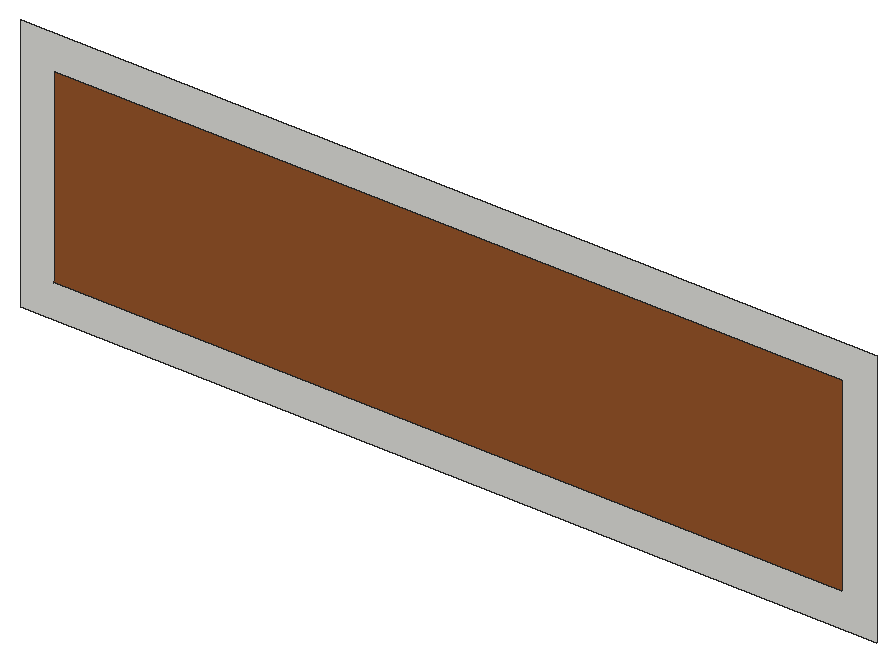
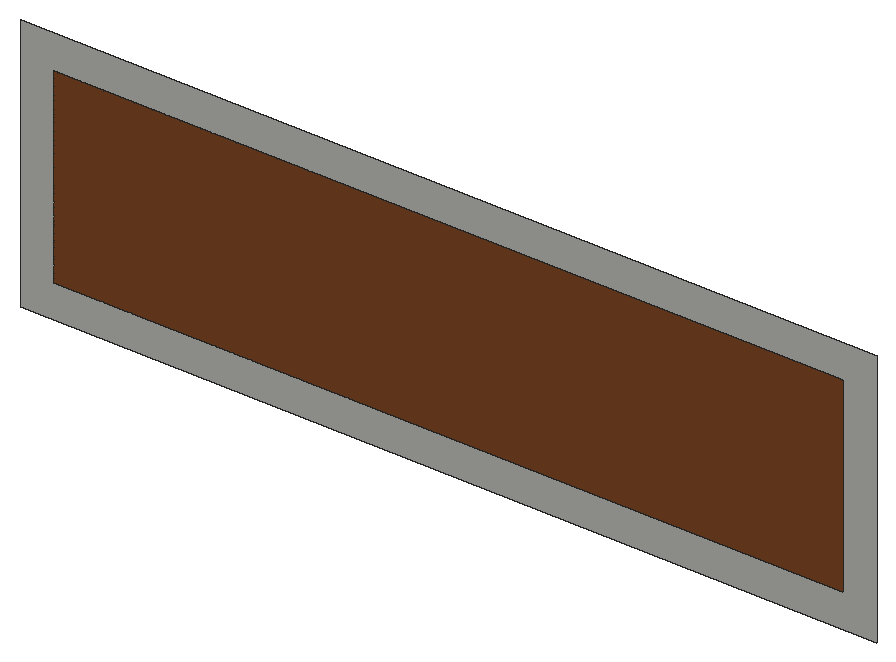
# SketchUp Ruby script. Lengths in inches.
U = 1.inch
M = Sketchup.active_model
def pt(a) = Geom::Point3d.new(a.map { |v| v * U })
def face(e, loops, mat)
  f = e.add_face(loops[0].map { |a| pt(a) })
  loops[1..].each { |l| e.add_face(l.map { |a| pt(a) }).erase! }
  f.material = f.back_material = mat if mat
  f
end
# faces: each face lists its corners as indices into pts; further lists are holes
def faces(e, pts, list, mat = nil) = list.each { |f| face(e, (f[0].is_a?(Array) ? f : [f]).map { |l| l.map { |i| pts[i] } }, mat) }
# xy, xz, yz: faces in a plane at the given z, y or x. An outline is a flat list of corners, or four numbers for a rectangle; further outlines are holes
def ring(l) = l.size == 4 ? [[l[0], l[1]], [l[2], l[1]], [l[2], l[3]], [l[0], l[3]]] : l.each_slice(2).to_a
def flat(e, list, mat, &to3) = list.each { |f| face(e, (f[0].is_a?(Array) ? f : [f]).map { |l| ring(l).map { |u, v| to3.(u, v) } }, mat) }
def xy(e, z, list, mat = nil) = flat(e, list, mat) { |x, y| [x, y, z] }
def xz(e, y, list, mat = nil) = flat(e, list, mat) { |x, z| [x, y, z] }
def yz(e, x, list, mat = nil) = flat(e, list, mat) { |y, z| [x, y, z] }
def lines(e, pts, list) = list.each { |a, b| e.add_line(pt(pts[a]), pt(pts[b])) }
# prism: a flat outline (further loops are holes) pulled along v
def prism(e, loops, v, mat = nil)
  f = face(e, loops, mat); d = Geom::Vector3d.new(v.map { |x| x * U })
  f.pushpull(f.normal.samedirection?(d) ? d.length : -d.length)
end
def box(e, o, s, mat = nil) = prism(e, [[o, [o[0] + s[0], o[1], o[2]], [o[0] + s[0], o[1] + s[1], o[2]], [o[0], o[1] + s[1], o[2]]]], [0, 0, s[2]], mat)
def at(x, y, z, deg = 0) = Geom::Transformation.translation(pt([x, y, z])) * Geom::Transformation.rotation(ORIGIN, Z_AXIS, deg.degrees)
def axes(o, x, y, z) = Geom::Transformation.new([*x, 0, *y, 0, *z, 0, *pt(o).to_a, 1])
def part(name) = M.definitions.add(name)
# library, detail: a bought-in or finely detailed component or shape, given as its bounding box
def library(name, o, s) = part(name).tap { |d| box(d.entities, o, s) }
def detail(e, o, s) = box(e.add_group.entities, o, s)
def put(e, d, t, mat = nil) = e.add_instance(d, t).tap { |i| i.material = mat if mat }
def group(e, t, mat = nil) = e.add_group.tap { |g| g.transformation = t; g.material = mat if mat }.entities
root = M.entities
M.materials.add("[Wood Cherry Original]1").color = [152, 86, 42]
xz(root,184.11,[[[341.12,39.83,445.24,71.08],[345.23,43.94,441.13,66.97]]])
xz(root,184.11,[[345.23,43.94,441.13,66.97]],"[Wood Cherry Original]1")
